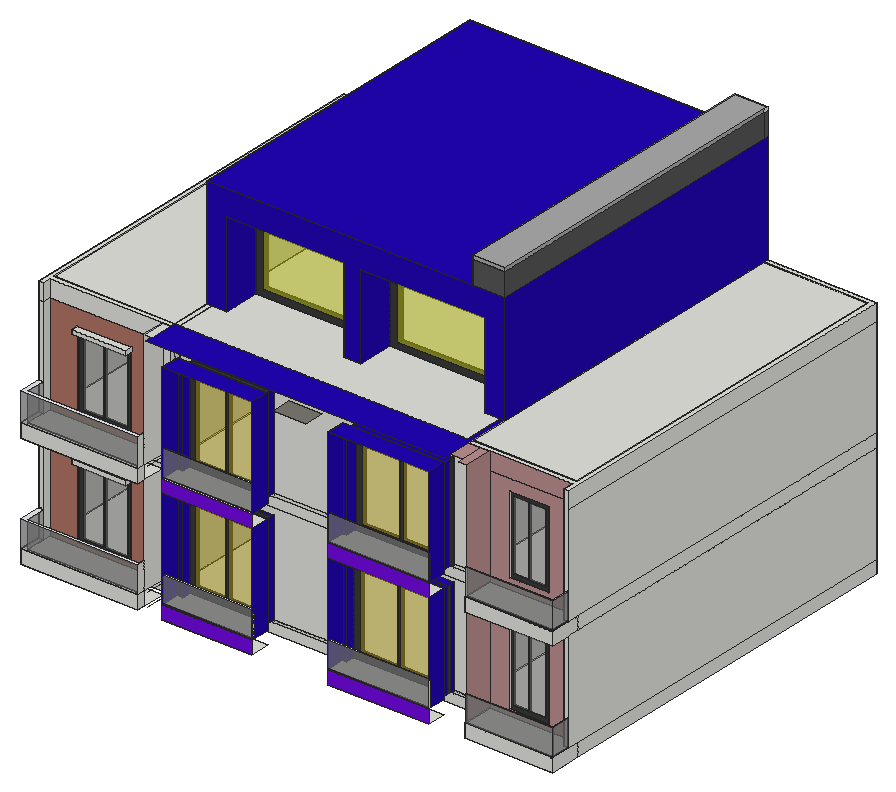
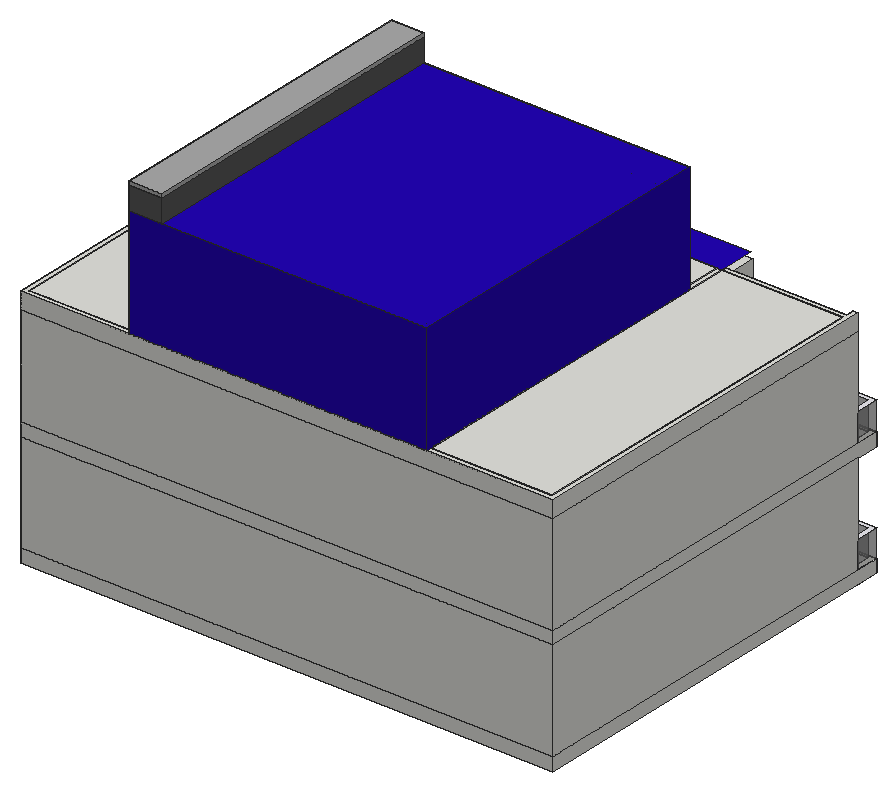
# SketchUp Ruby script. Lengths in inches.
U = 1.inch
M = Sketchup.active_model
def pt(a) = Geom::Point3d.new(a.map { |v| v * U })
def face(e, loops, mat)
  f = e.add_face(loops[0].map { |a| pt(a) })
  loops[1..].each { |l| e.add_face(l.map { |a| pt(a) }).erase! }
  f.material = f.back_material = mat if mat
  f
end
# faces: each face lists its corners as indices into pts; further lists are holes
def faces(e, pts, list, mat = nil) = list.each { |f| face(e, (f[0].is_a?(Array) ? f : [f]).map { |l| l.map { |i| pts[i] } }, mat) }
# xy, xz, yz: faces in a plane at the given z, y or x. An outline is a flat list of corners, or four numbers for a rectangle; further outlines are holes
def ring(l) = l.size == 4 ? [[l[0], l[1]], [l[2], l[1]], [l[2], l[3]], [l[0], l[3]]] : l.each_slice(2).to_a
def flat(e, list, mat, &to3) = list.each { |f| face(e, (f[0].is_a?(Array) ? f : [f]).map { |l| ring(l).map { |u, v| to3.(u, v) } }, mat) }
def xy(e, z, list, mat = nil) = flat(e, list, mat) { |x, y| [x, y, z] }
def xz(e, y, list, mat = nil) = flat(e, list, mat) { |x, z| [x, y, z] }
def yz(e, x, list, mat = nil) = flat(e, list, mat) { |y, z| [x, y, z] }
def lines(e, pts, list) = list.each { |a, b| e.add_line(pt(pts[a]), pt(pts[b])) }
# prism: a flat outline (further loops are holes) pulled along v
def prism(e, loops, v, mat = nil)
  f = face(e, loops, mat); d = Geom::Vector3d.new(v.map { |x| x * U })
  f.pushpull(f.normal.samedirection?(d) ? d.length : -d.length)
end
def box(e, o, s, mat = nil) = prism(e, [[o, [o[0] + s[0], o[1], o[2]], [o[0] + s[0], o[1] + s[1], o[2]], [o[0], o[1] + s[1], o[2]]]], [0, 0, s[2]], mat)
def at(x, y, z, deg = 0) = Geom::Transformation.translation(pt([x, y, z])) * Geom::Transformation.rotation(ORIGIN, Z_AXIS, deg.degrees)
def axes(o, x, y, z) = Geom::Transformation.new([*x, 0, *y, 0, *z, 0, *pt(o).to_a, 1])
def part(name) = M.definitions.add(name)
# library, detail: a bought-in or finely detailed component or shape, given as its bounding box
def library(name, o, s) = part(name).tap { |d| box(d.entities, o, s) }
def detail(e, o, s) = box(e.add_group.entities, o, s)
def put(e, d, t, mat = nil) = e.add_instance(d, t).tap { |i| i.material = mat if mat }
def group(e, t, mat = nil) = e.add_group.tap { |g| g.transformation = t; g.material = mat if mat }.entities
root = M.entities
M.materials.add("[0119_RosyBrown]").color = [188, 143, 143]
M.materials.add("[Brick Colored Blue]").color = [34, 5, 180]
M.materials.add("[Brick Colored Blue]1").color = [115, 11, 225]
M.materials.add("[Color M03]").color = [170, 170, 170]
M.materials.add("[Color M06]").color = [86, 86, 86]
M.materials.add("[Color M07]").color = [58, 58, 58]
M.materials.add("[Metal Silver]").color = [234, 233, 238]
M.materials.add("[Rough Square Concrete Block]").color = [123, 120, 113]
M.materials.add("[Stone Flagstone Ashlar]").color = [175, 116, 102]
M.materials.add("[Translucent Glass Blue]").color = [202, 178, 24]
M.materials["[Translucent Glass Blue]"].alpha = 0.5
M.materials.add("[Translucent Glass Blue]1").color = [227, 230, 22]
M.materials["[Translucent Glass Blue]1"].alpha = 0.5
M.materials.add("[Translucent Glass Gray]").color = [128, 128, 128]
M.materials["[Translucent Glass Gray]"].alpha = 0.5
c1 = part("Group\#2")
xy(c1.entities,0,[[0,0,124.375,6.5]],"[Color M07]")
xy(c1.entities,9.35,[[9.35,0,58.13,6.5],[62.66,0,115.02,6.5]],"[Color M07]")
xy(c1.entities,131.58,[[9.35,0,58.13,6.5],[62.66,0,115.02,6.5]],"[Color M07]")
xy(c1.entities,140.9375,[[0,0,124.375,6.5]],"[Color M07]")
xz(c1.entities,0,[[[0,0,124.375,140.9375],[62.66,9.35,115.02,131.58],[9.35,9.35,58.13,131.58]]],"[Color M07]")
xz(c1.entities,0,[[9.35,9.35,58.13,131.58],[62.66,9.35,115.02,131.58]],"[Translucent Glass Blue]")
xz(c1.entities,6.5,[[[0,0,124.375,140.9375],[62.66,9.35,115.02,131.58],[9.35,9.35,58.13,131.58]]],"[Color M07]")
yz(c1.entities,0,[[0,0,6.5,140.9375]],"[Color M07]")
yz(c1.entities,9.35,[[0,9.35,6.5,131.58]],"[Color M07]")
yz(c1.entities,58.13,[[0,9.35,6.5,131.58]],"[Color M07]")
yz(c1.entities,62.66,[[0,9.35,6.5,131.58]],"[Color M07]")
yz(c1.entities,115.02,[[0,9.35,6.5,131.58]],"[Color M07]")
yz(c1.entities,124.375,[[0,0,6.5,140.9375]],"[Color M07]")
c2 = part("Group\#1")
xy(c2.entities,0,[[0,0,103.0625,5.375]],"[Color M07]")
xy(c2.entities,8.61,[[8.61,0,48.54,5.375],[51.97,0,94.45,5.375]],"[Color M07]")
xy(c2.entities,158.15,[[8.61,0,48.54,5.375],[51.97,0,94.45,5.375]],"[Color M07]")
xy(c2.entities,166.76,[[0,0,103.0625,5.375]],"[Color M07]")
xz(c2.entities,0,[[[0,0,103.0625,166.76],[51.97,8.61,94.45,158.15],[8.61,8.61,48.54,158.15]]],"[Color M07]")
xz(c2.entities,0,[[8.61,8.61,48.54,158.15],[51.97,8.61,94.45,158.15]],"[Translucent Glass Gray]")
xz(c2.entities,5.375,[[[0,0,103.0625,166.76],[51.97,8.61,94.45,158.15],[8.61,8.61,48.54,158.15]]],"[Color M07]")
yz(c2.entities,0,[[0,0,5.375,166.76]],"[Color M07]")
yz(c2.entities,8.61,[[0,8.61,5.375,158.15]],"[Color M07]")
yz(c2.entities,48.54,[[0,8.61,5.375,158.15]],"[Color M07]")
yz(c2.entities,51.97,[[0,8.61,5.375,158.15]],"[Color M07]")
yz(c2.entities,94.45,[[0,8.61,5.375,158.15]],"[Color M07]")
yz(c2.entities,103.0625,[[0,0,5.375,166.76]],"[Color M07]")
c3 = part("Group\#3")
xy(c3.entities,0,[[0,0,167.1875,11.0625]],"[Color M07]")
xy(c3.entities,10.18,[[10.18,0,157.01,11.0625]],"[Color M07]")
xy(c3.entities,134.7,[[10.18,0,157.01,11.0625]],"[Color M07]")
xy(c3.entities,144.875,[[0,0,167.1875,11.0625]],"[Color M07]")
xz(c3.entities,0,[[[0,0,167.1875,144.875],[10.18,10.18,157.01,134.7]]],"[Color M07]")
xz(c3.entities,0,[[10.18,10.18,157.01,134.7]],"[Translucent Glass Blue]1")
xz(c3.entities,11.0625,[[[0,0,167.1875,144.875],[10.18,10.18,157.01,134.7]]],"[Color M07]")
yz(c3.entities,0,[[0,0,11.0625,144.875]],"[Color M07]")
yz(c3.entities,10.18,[[0,10.18,11.0625,134.7]],"[Color M07]")
yz(c3.entities,157.01,[[0,10.18,11.0625,134.7]],"[Color M07]")
yz(c3.entities,167.1875,[[0,0,11.0625,144.875]],"[Color M07]")
xy(root,600,[[0,110.3125,9,151.625],[9,110.3125,212.1875,166.4375],[255.8125,110.3125,417.96,145],[554.39,110.3125,736.375,145],[801.6875,110.3125,801.6875,166.4375,951,166.4375,951,147.0625,960,147.0625,960,110.3125]])
xy(root,618,[[9,175.4375,226.3125,831],[235.3125,175.4375,754.625,831],[763.625,175.4375,951,831]])
xy(root,624,[[0,110.3125,0,151.625,9,151.625,9,115.75,209.37,115.75,209.37,124.4375,212.1875,124.375,212.1875,110.3125],[255.8125,110.3125,417.96,111.625],[554.39,110.3125,736.375,111.625],[801.6875,110.3125,960,110.3125,960,147.0625,959.375,147.0625,959.375,111,801.6875,111],[801.6875,111,803.125,115.3125],
  [803.125,111,803.125,111.875,958.375,111.875,958.375,147.0625,959.375,147.0625,959.375,111],[255.8125,111.625,417.96,113.625],[554.39,111.625,736.375,113.625],[803.125,111.875,958.375,111.875,958.375,147.0625,951,147.0625,951,166.4375,801.6875,166.4375,801.6875,115.3125,803.125,115.3125],[255.8125,113.625,417.96,113.625,417.96,145,405.4,145,405.4,175.4375,265.83,175.4375,265.83,145,255.8125,145],
  [554.39,113.625,736.375,113.625,736.375,145,730.3125,145,730.3125,175.4375,560.75,175.4375,560.75,145,554.39,145],[9,115.75,209.37,115.75,209.37,124.4375,212.1875,124.375,212.1875,166.4375,9,166.4375],[9,175.4375,226.3125,831],[235.3125,175.4375,754.625,831],[763.625,175.4375,951,831]])
xy(root,629.71,[[59.43,166.4375,154.62,175.4375]])
xy(root,634.9,[[838.25,166.4375,907.94,175.4375]])
xy(root,672,[[803.125,111,959.375,111,959.375,147.0625,958.375,147.0625,958.375,111.875,803.125,111.875],[255.8125,111.625,417.96,113.625],[554.39,111.625,736.375,113.625]],"[Metal Silver]")
xy(root,672.6875,[[0,110.3125,212.1875,110.3125,212.1875,124.375,209.37,124.4375,209.37,115.75,9,115.75,9,151.625,0,151.625]],"[Metal Silver]")
xy(root,762.45,[[57.84,153.3125,57.84,166.4375,59.43,166.4375,59.43,175.4375,154.62,175.4375,154.62,166.4375,155.9,166.4375,155.9,153.3125]])
xy(root,770.35,[[57.84,153.3125,155.9,166.4375]])
xy(root,775.28,[[838.25,166.4375,907.94,175.4375]])
xy(root,792.31,[[265.83,145,405.4,175.4375]],"[Brick Colored Blue]")
xy(root,798.35,[[560.75,145,730.3125,175.4375]],"[Brick Colored Blue]")
xy(root,804,[[0,110.3125,9,151.625],[9,110.3125,212.1875,166.4375],[255.8125,110.3125,417.96,145],[554.39,110.3125,736.375,145],[801.6875,110.3125,801.6875,166.4375,951,166.4375,951,147.0625,960,147.0625,960,110.3125]])
xy(root,822,[[9,175.4375,226.3125,831],[235.3125,175.4375,754.625,831],[763.625,175.4375,951,831]])
xy(root,828,[[0,110.3125,0,151.625,9,151.625,9,116.6875,209.9375,116.6875,209.9375,124.4375,212.1875,124.4375,212.1875,110.3125],[255.8125,110.3125,417.96,111.875],[554.39,110.3125,736.375,111.875],[801.6875,110.3125,960,110.3125,960,147.0625,959.25,147.0625,959.25,111.6875,801.6875,111.6875],[801.6875,111.6875,802.5625,115.3125],
  [802.5625,111.6875,802.5625,113.6875,957.5625,113.6875,957.5625,147.0625,959.25,147.0625,959.25,111.6875],[554.39,111.875,736.375,113.875],[802.5625,113.6875,957.5625,113.6875,957.5625,147.0625,951,147.0625,951,166.4375,801.6875,166.4375,801.6875,115.3125,802.5625,115.3125],[255.8125,113.875,417.96,113.875,417.96,145,405.4,145,405.4,175.4375,265.83,175.4375,265.83,145,255.8125,145],[554.39,113.875,736.375,113.875,736.375,145,730.3125,145,730.3125,175.4375,560.75,175.4375,560.75,145,554.39,145],
  [9,116.6875,209.9375,116.6875,209.9375,124.4375,212.1875,124.4375,212.1875,166.4375,9,166.4375],[9,175.4375,226.3125,831],[235.3125,175.4375,754.625,831],[763.625,175.4375,951,831]])
xy(root,839.33,[[59.43,166.4375,154.62,175.4375]])
xy(root,847.47,[[838.25,166.4375,907.94,175.4375]])
xy(root,876,[[802.5625,111.6875,959.25,111.6875,959.25,147.0625,957.5625,147.0625,957.5625,113.6875,802.5625,113.6875],[255.8125,111.875,417.96,113.875],[554.39,111.875,736.375,113.875]],"[Metal Silver]")
xy(root,879.5,[[0,110.3125,212.1875,110.3125,212.1875,124.4375,209.9375,124.4375,209.9375,116.6875,9,116.6875,9,151.625,0,151.625]],"[Metal Silver]")
xy(root,972.07,[[57.84,153.75,57.84,166.4375,59.43,166.4375,59.43,175.4375,154.62,175.4375,154.62,166.4375,155.9,166.4375,155.9,153.75]])
xy(root,979.97,[[57.84,153.75,155.9,166.4375]])
xy(root,987.84,[[838.25,166.4375,907.94,175.4375]])
xy(root,997.43,[[265.83,145,405.4,175.4375]],"[Brick Colored Blue]")
xy(root,998.875,[[763.625,175.4375,951,831]])
xy(root,1000.29,[[560.75,145,730.3125,175.4375]],"[Brick Colored Blue]")
xy(root,1008,[[255.8125,110.3125,417.96,145],[554.39,110.3125,736.375,145]],"[Brick Colored Blue]")
xy(root,1008,[[456.7,110.3125,515.65,145]],"[Rough Square Concrete Block]")
xy(root,1033.1875,[[9,175.4375,226.3125,831],[235.3125,175.4375,754.625,831]])
xy(root,1039.1875,[[212.1875,124.375,226.3125,166.4375],[951,147.0625,960,147.0625,960,840,763.625,840,763.625,831,951,831,951,175.4375,763.625,175.4375,763.625,166.4375,951,166.4375],[0,151.625,9,151.625,9,166.4375,226.3125,166.4375,226.3125,175.4375,235.3125,175.4375,235.3125,248.5,226.3125,248.5,226.3125,175.4375,9,175.4375,9,831,226.3125,831,226.3125,840,0,840],[9,175.4375,226.3125,831],[235.3125,175.4375,754.625,175.4375,754.625,248.5,727.75,248.5,727.75,314.25,503.82,314.25,503.82,248.5,471.99,248.5,471.99,314.25,262.4375,314.25,262.4375,248.5,235.3125,248.5],
  [763.625,175.4375,951,831],[226.3125,248.5,226.3125,840,763.625,840,763.625,248.5,754.625,248.5,754.625,831,235.3125,831,235.3125,248.5],[235.3125,248.5,262.4375,256.71],[471.99,248.5,503.82,314.25],[727.75,248.5,754.625,267.5625],
  [235.3125,256.71,262.4375,267.5625],[235.3125,267.5625,262.4375,314.25],[727.75,267.5625,754.625,314.25],[235.3125,314.25,754.625,831]])
xy(root,1039.1875,[[786.375,115.3125,801.6875,166.4375],[763.625,124.625,786.375,166.4375]],"[0119_RosyBrown]")
xy(root,1039.1875,[[226.3125,110.3125,763.625,110.3125,763.625,248.5,754.625,248.5,754.625,175.4375,226.3125,175.4375]],"[Brick Colored Blue]")
xy(root,1191.81,[[262.4375,248.5,471.99,314.25],[503.82,248.5,727.75,314.25]])
xy(root,1214.875,[[235.3125,314.25,754.625,831]])
xy(root,1219.1875,[[235.3125,314.25,754.625,831]])
xy(root,1232.625,[[235.3125,314.25,754.625,831]])
xy(root,1237.625,[[704.99,248.5,763.625,840]])
xy(root,1237.625,[[226.3125,248.5,704.99,840]],"[Brick Colored Blue]")
xy(root,1279.9375,[[704.99,248.5,763.625,840]])
xy(root,1286.1875,[[704.99,248.5,763.625,840]],"[Color M03]")
xz(root,110.3125,[[0,600,212.1875,624],[801.6875,600,960,624],[0,804,212.1875,828],[801.6875,804,960,828]])
xz(root,110.3125,[[255.8125,600,417.96,624],[554.39,600,736.375,624],[255.8125,804,417.96,828],[554.39,804,736.375,828]],"[Brick Colored Blue]1")
xz(root,110.3125,[[0,624,212.1875,672.6875],[0,828,212.1875,879.5]],"[Translucent Glass Gray]")
xz(root,111,[[959.1875,624,959.375,672]])
xz(root,111,[[803.125,624,959.1875,672]],"[Translucent Glass Gray]")
xz(root,111.625,[[255.8125,624,417.96,672],[554.39,624,736.375,672]],"[Translucent Glass Gray]")
xz(root,111.6875,[[802.5625,828,959.25,876]],"[Translucent Glass Gray]")
xz(root,111.875,[[803.125,624,958.375,672],[255.8125,828,417.96,876],[554.39,828,736.375,876]],"[Translucent Glass Gray]")
xz(root,113.625,[[255.8125,624,417.96,672],[554.39,624,736.375,672]],"[Translucent Glass Gray]")
xz(root,113.6875,[[802.5625,828,957.5625,876]],"[Translucent Glass Gray]")
xz(root,113.875,[[255.8125,828,417.96,876],[554.39,828,736.375,876]],"[Translucent Glass Gray]")
xz(root,115.75,[[9,624,209.37,672.6875]],"[Translucent Glass Gray]")
xz(root,116.6875,[[9,828,209.9375,879.5]],"[Translucent Glass Gray]")
xz(root,124.4375,[[209.9375,828,212.1875,879.5]])
xz(root,145,[[255.8125,624,265.83,624,265.83,792.31,405.4,792.31,405.4,624,417.96,624,417.96,804,255.8125,804],[554.39,624,560.75,624,560.75,798.35,730.3125,798.35,730.3125,624,736.375,624,736.375,804,554.39,804],[255.8125,828,265.83,828,265.83,997.43,405.4,997.43,405.4,828,417.96,828,417.96,1008,255.8125,1008],[554.39,828,560.75,828,560.75,1000.29,730.3125,1000.29,730.3125,828,736.375,828,736.375,1008,554.39,1008]],"[Brick Colored Blue]")
xz(root,147.0625,[[951,624,958.375,624,958.375,672,959.375,672,959.375,624,960,624,960,804,951,804],[958.375,624,959.375,672],[951,828,957.5625,828,957.5625,876,959.25,876,959.25,828,960,828,960,1039.1875,951,1039.1875],[957.5625,828,959.25,876]])
xz(root,151.625,[[2.54,616.14,6.79,620.39],[0,624,9,672],[0,672,9,672.6875],[0,672.6875,9,804],[0,828,9,876],
  [0,876,9,879.5],[0,879.5,9,1008],[0,1008,9,1039.1875]])
xz(root,153.3125,[[57.84,762.45,155.9,770.35]])
xz(root,153.75,[[57.84,972.07,155.9,979.97]])
xz(root,166.4375,[[217.1875,600,226.3125,624],[763.625,600,786.375,624],[786.375,600,801.6875,624],[212.1875,624,226.3125,804],[763.625,624,786.375,804],
  [786.375,624,801.6875,804],[217.1875,804,226.3125,828],[763.625,804,786.375,828],[786.375,804,801.6875,828],[212.1875,828,226.3125,1008],
  [763.625,828,786.375,1008],[786.375,828,801.6875,1008],[9,1008,212.1875,1039.1875],[212.1875,1008,226.3125,1039.1875],[763.625,1008,786.375,1039.1875],
  [786.375,1008,801.6875,1039.1875]])
xz(root,166.4375,[[[801.6875,624,951,804],[838.25,634.9,907.94,775.28]],[[801.6875,828,951,1008],[838.25,847.47,907.94,987.84]],[801.6875,1008,951,1039.1875]],"[0119_RosyBrown]")
xz(root,166.4375,[[[9,624,212.1875,804],[59.43,629.71,59.43,762.45,57.84,762.45,57.84,770.35,155.9,770.35,155.9,762.45,154.62,762.45,154.62,629.71]],[[9,828,212.1875,1008],[59.43,839.33,59.43,972.07,57.84,972.07,57.84,979.97,155.9,979.97,155.9,972.07,154.62,972.07,154.62,839.33]]],"[Stone Flagstone Ashlar]")
xz(root,175.4375,[[9,600,226.3125,618],[235.3125,600,754.625,618],[763.625,600,951,618],[9,618,226.3125,624],[235.3125,618,265.83,624],
  [265.83,618,405.4,624],[405.4,618,560.75,624],[560.75,618,730.3125,624],[730.3125,618,754.625,624],[763.625,618,951,624],
  [[9,624,226.3125,804],[59.43,629.71,154.62,762.45]],[235.3125,624,235.3125,804,754.625,804,754.625,624,730.3125,624,730.3125,798.35,560.75,798.35,560.75,624,405.4,624,405.4,792.31,265.83,792.31,265.83,624],[[763.625,624,951,804],[838.25,634.9,907.94,775.28]],[9,804,226.3125,822],[235.3125,804,754.625,822],
  [763.625,804,951,822],[9,822,226.3125,828],[235.3125,822,265.83,828],[265.83,822,405.4,828],[405.4,822,560.75,828],
  [560.75,822,730.3125,828],[730.3125,822,754.625,828],[763.625,822,951,828],[[9,828,226.3125,1008],[59.43,839.33,154.62,972.07]],[235.3125,828,235.3125,1008,754.625,1008,754.625,828,730.3125,828,730.3125,1000.29,560.75,1000.29,560.75,828,405.4,828,405.4,997.43,265.83,997.43,265.83,828],
  [[763.625,828,951,998.875],[838.25,847.47,907.94,987.84]],[763.625,998.875,951,1008],[9,1008,226.3125,1033.1875],[235.3125,1008,754.625,1033.1875],[763.625,1008,951,1039.1875],
  [9,1033.1875,226.3125,1039.1875],[235.3125,1033.1875,754.625,1039.1875]])
xz(root,248.5,[[226.3125,1039.1875,262.4375,1039.1875,262.4375,1191.81,471.99,1191.81,471.99,1039.1875,503.82,1039.1875,503.82,1191.81,727.75,1191.81,727.75,1039.1875,763.625,1039.1875,763.625,1237.625,226.3125,1237.625]],"[Brick Colored Blue]")
xz(root,248.5,[[704.99,1279.9375,763.625,1286.1875]],"[Color M03]")
xz(root,248.5,[[704.99,1237.625,763.625,1279.9375]],"[Color M06]")
xz(root,267.5625,[[727.75,1039.1875,754.625,1191.81]])
xz(root,314.25,[[235.3125,1039.1875,235.3125,1214.875,754.625,1214.875,754.625,1039.1875,727.75,1039.1875,727.75,1191.81,503.82,1191.81,503.82,1039.1875,471.99,1039.1875,471.99,1191.81,262.4375,1191.81,262.4375,1039.1875],[235.3125,1214.875,238.4375,1219.1875],[238.4375,1214.875,754.625,1219.1875],[235.3125,1219.1875,238.4375,1232.625],[238.4375,1219.1875,754.625,1232.625]])
xz(root,831,[[9,600,226.3125,618],[235.3125,600,754.625,618],[763.625,600,951,618],[9,618,226.3125,624],[235.3125,618,754.625,624],
  [763.625,618,824.65,624],[824.65,618,839.21,624],[839.21,618,951,624],[9,624,226.3125,804],[235.3125,624,754.625,804],
  [763.625,624,951,804],[9,804,226.3125,822],[235.3125,804,754.625,822],[763.625,804,951,822],[9,822,226.3125,828],
  [235.3125,822,754.625,828],[763.625,822,857.3125,828],[857.3125,822,873,828],[873,822,951,828],[9,828,226.3125,1008],
  [235.3125,828,754.625,1008],[763.625,828,951,998.875],[763.625,998.875,904.38,1008],[904.38,998.875,915.19,1008],[915.19,998.875,951,1008],
  [9,1008,226.3125,1033.1875],[235.3125,1008,754.625,1033.1875],[763.625,1008,904.38,1039.1875],[904.38,1008,915.19,1039.1875],[915.19,1008,951,1039.1875],
  [9,1033.1875,226.3125,1039.1875],[235.3125,1033.1875,754.625,1039.1875],[235.3125,1039.1875,754.625,1214.875],[235.3125,1214.875,754.625,1219.1875],[235.3125,1219.1875,754.625,1232.625]])
xz(root,840,[[0,600,960,624],[0,624,960,804],[0,804,960,828],[0,828,960,1008],[0,1008,960,1039.1875]])
xz(root,840,[[226.3125,1039.1875,763.625,1237.625]],"[Brick Colored Blue]")
xz(root,840,[[704.99,1279.9375,763.625,1286.1875]],"[Color M03]")
xz(root,840,[[704.99,1237.625,763.625,1279.9375]],"[Color M06]")
yz(root,0,[[110.3125,600,840,624],[151.625,624,840,804],[110.3125,804,840,828],[151.625,828,840,1008],[151.625,1008,840,1039.1875]])
yz(root,0,[[110.3125,624,151.625,672.6875],[110.3125,828,151.625,879.5]],"[Translucent Glass Gray]")
yz(root,9,[[175.4375,600,831,618],[175.4375,618,269.47,624],[269.47,618,281.72,624],[281.72,618,831,624],[151.625,624,166.4375,804],
  [175.4375,624,831,804],[175.4375,804,831,822],[175.4375,822,330.46,828],[330.46,822,340.84,828],[340.84,822,831,828],
  [151.625,828,166.4375,1008],[175.4375,828,831,1008],[151.625,1008,166.4375,1039.1875],[175.4375,1008,831,1033.1875],[175.4375,1033.1875,269.47,1039.1875],
  [269.47,1033.1875,301.78,1039.1875],[301.78,1033.1875,831,1039.1875]])
yz(root,9,[[115.75,624,151.625,672.6875],[116.6875,828,151.625,879.5]],"[Translucent Glass Gray]")
yz(root,57.84,[[153.3125,762.45,166.4375,770.35],[153.75,972.07,166.4375,979.97]])
yz(root,59.43,[[166.4375,629.71,175.4375,762.45],[166.4375,839.33,175.4375,972.07]])
yz(root,154.62,[[166.4375,629.71,175.4375,762.45],[166.4375,839.33,175.4375,972.07]])
yz(root,155.9,[[153.3125,762.45,166.4375,770.35],[153.75,972.07,166.4375,979.97]])
yz(root,209.37,[[115.75,624,124.4375,672.6875]])
yz(root,209.9375,[[116.6875,828,124.4375,879.5]])
yz(root,212.1875,[[110.3125,600,124.375,624],[110.3125,624,124.375,672.6875],[124.375,624,166.4375,804],[110.3125,804,124.375,828],[110.3125,828,124.375,879.5],
  [124.375,828,124.4375,879.5],[124.4375,828,124.4375,879.5,124.375,879.5,124.375,1039.1875,166.4375,1039.1875,166.4375,828]])
yz(root,226.3125,[[166.4375,600,175.4375,624],[175.4375,600,831,618],[175.4375,618,831,624],[166.4375,624,175.4375,804],[175.4375,624,831,804],
  [166.4375,804,175.4375,828],[175.4375,804,831,822],[175.4375,822,831,828],[166.4375,828,175.4375,1008],[175.4375,828,831,1008],
  [166.4375,1008,175.4375,1039.1875],[175.4375,1008,831,1033.1875],[175.4375,1033.1875,831,1039.1875]])
yz(root,226.3125,[[248.5,1039.1875,840,1237.625]],"[Brick Colored Blue]")
yz(root,235.3125,[[175.4375,600,831,618],[175.4375,618,244.42,624],[244.42,618,256.71,624],[256.71,618,831,624],[175.4375,624,831,804],
  [175.4375,804,831,822],[175.4375,822,216.11,828],[216.11,822,230.67,828],[230.67,822,831,828],[175.4375,828,831,1008],
  [175.4375,1008,831,1033.1875],[175.4375,1033.1875,256.71,1039.1875],[256.71,1033.1875,274.65,1039.1875],[274.65,1033.1875,831,1039.1875],[314.25,1039.1875,831,1214.875],
  [314.25,1214.875,831,1219.1875],[314.25,1219.1875,831,1232.625]])
yz(root,255.8125,[[111.625,624,113.625,672]])
yz(root,255.8125,[[110.3125,624,111.625,624,111.625,672,113.625,672,113.625,624,145,624,145,804,110.3125,804],[110.3125,828,111.875,828,111.875,876,113.875,876,113.875,828,145,828,145,1008,110.3125,1008]],"[Brick Colored Blue]")
yz(root,262.4375,[[248.5,1039.1875,314.25,1191.81]],"[Brick Colored Blue]")
yz(root,265.83,[[145,624,175.4375,792.31],[145,828,175.4375,997.43]],"[Brick Colored Blue]")
yz(root,405.4,[[145,624,175.4375,792.31],[145,828,175.4375,997.43]],"[Brick Colored Blue]")
yz(root,417.96,[[111.625,624,113.625,672]])
yz(root,417.96,[[110.3125,624,110.3125,804,145,804,145,624,113.625,624,113.625,672,111.625,672,111.625,624],[110.3125,828,110.3125,1008,145,1008,145,828,113.875,828,113.875,876,111.875,876,111.875,828]],"[Brick Colored Blue]")
yz(root,471.99,[[248.5,1039.1875,314.25,1191.81]],"[Brick Colored Blue]")
yz(root,503.82,[[248.5,1039.1875,314.25,1191.81]],"[Brick Colored Blue]")
yz(root,554.39,[[111.625,624,113.625,672],[111.875,828,113.875,876]])
yz(root,554.39,[[110.3125,624,111.625,624,111.625,672,113.625,672,113.625,624,145,624,145,804,110.3125,804],[110.3125,828,111.875,828,111.875,876,113.875,876,113.875,828,145,828,145,1008,110.3125,1008]],"[Brick Colored Blue]")
yz(root,560.75,[[145,624,175.4375,798.35],[145,828,175.4375,1000.29]],"[Brick Colored Blue]")
yz(root,704.99,[[248.5,1279.9375,840,1286.1875]],"[Color M03]")
yz(root,704.99,[[248.5,1237.625,840,1279.9375]],"[Color M06]")
yz(root,727.75,[[248.5,1039.1875,267.5625,1191.81],[267.5625,1039.1875,314.25,1191.81]],"[Brick Colored Blue]")
yz(root,730.3125,[[145,624,175.4375,798.35],[145,828,175.4375,1000.29]],"[Brick Colored Blue]")
yz(root,736.375,[[111.625,624,113.625,672],[111.875,828,113.875,876]])
yz(root,736.375,[[110.3125,624,110.3125,804,145,804,145,624,113.625,624,113.625,672,111.625,672,111.625,624],[110.3125,828,110.3125,1008,145,1008,145,828,113.875,828,113.875,876,111.875,876,111.875,828]],"[Brick Colored Blue]")
yz(root,754.625,[[175.4375,600,831,618],[175.4375,618,831,624],[175.4375,624,831,804],[175.4375,804,831,822],[175.4375,822,831,828],
  [175.4375,828,831,1008],[175.4375,1008,831,1033.1875],[175.4375,1033.1875,831,1039.1875],[314.25,1039.1875,831,1214.875],[314.25,1214.875,831,1219.1875],
  [314.25,1219.1875,831,1232.625]])
yz(root,763.625,[[166.4375,600,175.4375,624],[175.4375,600,831,618],[175.4375,618,831,624],[166.4375,624,175.4375,804],[175.4375,624,831,804],
  [166.4375,804,175.4375,828],[175.4375,804,831,822],[175.4375,822,831,828],[166.4375,828,175.4375,1008],[175.4375,828,831,998.875],
  [175.4375,998.875,831,1008],[166.4375,1008,175.4375,1039.1875],[175.4375,1008,831,1039.1875],[831,1279.9375,840,1286.1875]])
yz(root,763.625,[[248.5,1039.1875,840,1237.625]],"[Brick Colored Blue]")
yz(root,763.625,[[248.5,1279.9375,831,1286.1875]],"[Color M03]")
yz(root,763.625,[[248.5,1237.625,831,1279.9375],[831,1237.625,840,1279.9375]],"[Color M06]")
yz(root,801.6875,[[110.3125,600,115.3125,624],[115.3125,600,166.4375,624],[110.3125,804,115.3125,828],[115.3125,804,166.4375,828]])
yz(root,801.6875,[[115.3125,624,166.4375,804],[115.3125,828,166.4375,1039.1875]],"[0119_RosyBrown]")
yz(root,802.5625,[[111.6875,828,113.6875,876]])
yz(root,803.125,[[111,624,111.875,672]])
yz(root,838.25,[[166.4375,634.9,175.4375,775.28],[166.4375,847.47,175.4375,987.84]])
yz(root,907.94,[[166.4375,634.9,175.4375,775.28],[166.4375,847.47,175.4375,987.84]])
yz(root,951,[[175.4375,600,831,618],[175.4375,618,831,624],[147.0625,624,166.4375,804],[175.4375,624,831,804],[175.4375,804,831,822],
  [175.4375,822,831,828],[147.0625,828,166.4375,1008],[175.4375,828,831,998.875],[175.4375,998.875,831,1008],[147.0625,1008,166.4375,1039.1875],
  [175.4375,1008,831,1039.1875]])
yz(root,957.5625,[[113.6875,828,147.0625,876]],"[Translucent Glass Gray]")
yz(root,958.375,[[111.875,624,147.0625,672]],"[Translucent Glass Gray]")
yz(root,959.25,[[111.6875,828,147.0625,876]],"[Translucent Glass Gray]")
yz(root,959.375,[[111,624,147.0625,672]],"[Translucent Glass Gray]")
yz(root,960,[[110.3125,600,166.4375,624],[166.4375,600,840,624],[147.0625,624,840,804],[110.3125,804,166.4375,828],[166.4375,804,840,828],
  [147.0625,828,840,1008],[147.0625,1008,840,1039.1875]])
p = [[212.1875,124.375,624],[209.37,124.4375,624],[209.37,124.4375,672.6875],[212.1875,124.375,672.6875],[217.1875,166.4375,828],[217.1875,124.375,828],
  [217.1875,166.4375,600],[217.1875,124.375,600],[217.1875,166.4375,624],[217.1875,124.375,624],[754.625,267.5625,1191.81],[754.625,248.5,1191.81],
  [279.375,314.25,1237.625],[279.375,314.25,1232.625],[235.3125,831,1232.625],[235.3125,831,1237.625],[754.625,314.25,1232.625],[754.625,314.25,1237.625],
  [235.3125,314.25,1232.625],[235.3125,314.25,1237.625]]
faces(root,p,[[0,1,2,3]])
lines(root,p,[[4,5],[6,7],[8,9],[10,11],[12,13],[14,15],[16,17],[18,19]])
put(root,c1,axes([560.75,160.22,624],[1.36332,0,0],[0,1,0],[0,0,1.23706]))
put(root,c1,axes([265.83,160.22,625.125],[1.12211,0,0],[0,1,0],[0,0,1.20218]))
put(root,c2,axes([59.43,168.32,629.71],[0.92359,0,0],[0,0.65,0],[0,0,0.796]))
put(root,c2,axes([838.25,167.89,634.9],[0.67617,0,0],[0,0.325,0],[0,0,0.84179]))
put(root,c1,axes([265.83,160.22,828],[1.12211,0,0],[0,1,0],[0,0,1.20218]))
put(root,c1,axes([560.75,166.1875,828],[1.36332,0,0],[0,1,0],[0,0,1.22243]))
put(root,c2,axes([59.43,168.32,839.33],[0.92359,0,0],[0,0.65,0],[0,0,0.796]))
put(root,c2,axes([838.25,167.89,847.47],[0.67617,0,0],[0,0.325,0],[0,0,0.84179]))
put(root,c3,axes([262.4375,314.25,1039.1875],[1.25338,0,0],[0,1,0],[0,0,1.05347]))
put(root,c3,axes([503.82,314.25,1039.1875],[1.33938,0,0],[0,1,0],[0,0,1.05347]))
